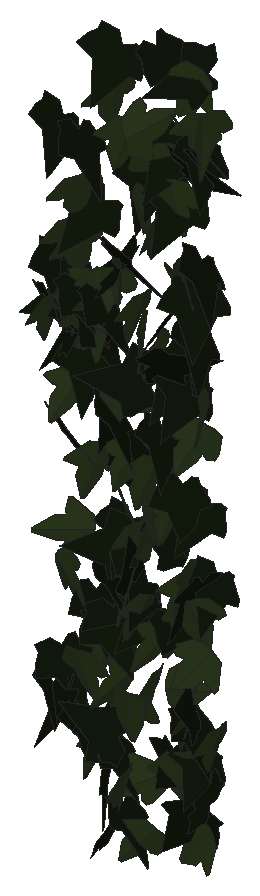
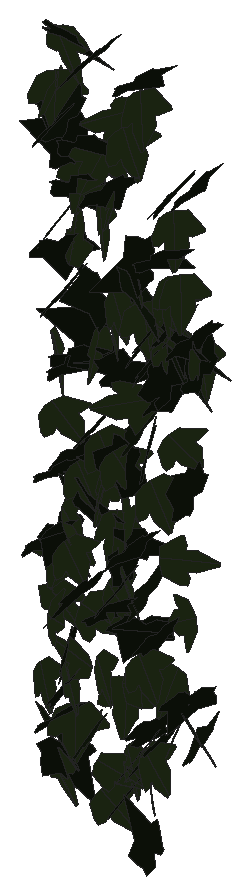
# SketchUp Ruby script. Lengths in inches.
U = 1.inch
M = Sketchup.active_model
def pt(a) = Geom::Point3d.new(a.map { |v| v * U })
def face(e, loops, mat)
  f = e.add_face(loops[0].map { |a| pt(a) })
  loops[1..].each { |l| e.add_face(l.map { |a| pt(a) }).erase! }
  f.material = f.back_material = mat if mat
  f
end
# faces: each face lists its corners as indices into pts; further lists are holes
def faces(e, pts, list, mat = nil) = list.each { |f| face(e, (f[0].is_a?(Array) ? f : [f]).map { |l| l.map { |i| pts[i] } }, mat) }
# xy, xz, yz: faces in a plane at the given z, y or x. An outline is a flat list of corners, or four numbers for a rectangle; further outlines are holes
def ring(l) = l.size == 4 ? [[l[0], l[1]], [l[2], l[1]], [l[2], l[3]], [l[0], l[3]]] : l.each_slice(2).to_a
def flat(e, list, mat, &to3) = list.each { |f| face(e, (f[0].is_a?(Array) ? f : [f]).map { |l| ring(l).map { |u, v| to3.(u, v) } }, mat) }
def xy(e, z, list, mat = nil) = flat(e, list, mat) { |x, y| [x, y, z] }
def xz(e, y, list, mat = nil) = flat(e, list, mat) { |x, z| [x, y, z] }
def yz(e, x, list, mat = nil) = flat(e, list, mat) { |y, z| [x, y, z] }
def lines(e, pts, list) = list.each { |a, b| e.add_line(pt(pts[a]), pt(pts[b])) }
# prism: a flat outline (further loops are holes) pulled along v
def prism(e, loops, v, mat = nil)
  f = face(e, loops, mat); d = Geom::Vector3d.new(v.map { |x| x * U })
  f.pushpull(f.normal.samedirection?(d) ? d.length : -d.length)
end
def box(e, o, s, mat = nil) = prism(e, [[o, [o[0] + s[0], o[1], o[2]], [o[0] + s[0], o[1] + s[1], o[2]], [o[0], o[1] + s[1], o[2]]]], [0, 0, s[2]], mat)
def at(x, y, z, deg = 0) = Geom::Transformation.translation(pt([x, y, z])) * Geom::Transformation.rotation(ORIGIN, Z_AXIS, deg.degrees)
def axes(o, x, y, z) = Geom::Transformation.new([*x, 0, *y, 0, *z, 0, *pt(o).to_a, 1])
def part(name) = M.definitions.add(name)
# library, detail: a bought-in or finely detailed component or shape, given as its bounding box
def library(name, o, s) = part(name).tap { |d| box(d.entities, o, s) }
def detail(e, o, s) = box(e.add_group.entities, o, s)
def put(e, d, t, mat = nil) = e.add_instance(d, t).tap { |i| i.material = mat if mat }
def group(e, t, mat = nil) = e.add_group.tap { |g| g.transformation = t; g.material = mat if mat }.entities
root = M.entities
M.materials.add("efeu1").color = [18, 25, 13]
M.materials.add("efeu2").color = [43, 57, 29]
c1 = part("ivyleaf_10")
p = [[0,0.5,-0.03],[-0.0625,2.02,-0.43],[-0.19,2.01,-0.46],[-0.54,1.05,-0.29],[-0.52,0.625,-0.18],[-0.83,0.76,-0.28],
  [-1.16,0.64,-0.33],[-1.15,0.33,-0.24],[-0.77,-0.39,0.02],[-0.3,-0.51,0.16],[0.04,-0.48,0.23],[-0.02,2.01,-0.4375],
  [-0.06,2.01,-0.43],[0.04,-0.49,0.23],[0.67,-0.49,0.14],[1.38,0.36,-0.2],[1.375,0.51,-0.24],[0.81,0.65,-0.19],
  [0.62,0.59,-0.15],[0.6,1.09,-0.28],[0.5,1.23,-0.31]]
faces(c1.entities,p,[[0,1,2,3,4,5,6,7,8,9,10],[11,12,0,13,14,15,16,17,18,19,20]],"efeu2")
c2 = part("ivyleaf_9")
p = [[1.54,2.16,1.25],[1.36,2.04,1.19],[-0.21,0.99,0.68],[-0.71,1.11,0.82],[-0.85,0.86,0.67],[-0.8,0.17,0.21],
  [-0.9,-0.01,0.1],[-0.67,-0.16,-0.02],[-0.08,-0.08,-0.05],[-0.03,-0.6,-0.4],[0.65,-0.88,-0.66],[0.83,-0.6,-0.49],
  [1.29,-0.42,-0.43],[1.8125,-0.07,-0.26],[1.21,0.44,0.15]]
faces(c2.entities,p,[[0,1,2,3,4,5,6,7,8,9,10,11,12,13,14]],"efeu1")
put(root,c1,axes([535.13,131.05,220.32],[0.3566,-0.77108,0.40331],[0.15176,-0.37408,-0.84937],[0.85685,0.38716,-0.01742]))
put(root,c2,axes([529.67,130.77,229.66],[-0.79255,0.50214,-0.23003],[0.19166,-0.12729,-0.93823],[-0.518,-0.81539,0.0048]))
put(root,c2,axes([529.14,130.89,212.83],[-0.83866,0.25323,-0.33738],[0.32395,-0.0943,-0.87605],[-0.2702,-0.89905,-0.00314]))
put(root,c2,axes([532.88,131.13,227.81],[-0.47309,-0.04164,0.86043],[-0.83764,-0.20693,-0.47057],[0.2011,-0.95986,0.06412]))
put(root,c1,axes([533.75,130.17,222.83],[-0.46435,0.56277,0.68264],[-0.40566,0.54969,-0.72911],[-0.78622,-0.616,-0.02698]))
put(root,c1,axes([529.6,131.16,220.19],[-0.05392,0.07152,0.95533],[-0.66511,-0.69145,0.01423],[0.68949,-0.66141,0.08843]))
put(root,c1,axes([528.33,130.79,230.19],[0.02915,-0.97812,-0.05689],[-0.00777,0.05668,-0.97854],[0.97974,0.02955,-0.00607]))
put(root,c2,axes([535.57,131.06,233],[-0.44583,-0.80919,-0.30244],[0.12747,0.275,-0.92366],[0.85441,-0.46326,-0.02002]))
put(root,c1,axes([533.64,130.37,222.18],[0.08945,-0.72433,-0.6179],[0.01533,0.62164,-0.72649],[0.95196,0.05805,0.06976]))
put(root,c1,axes([531.99,130.83,209.91],[0.21532,-0.88459,-0.06379],[-0.01557,0.06186,-0.91042],[0.88675,0.21588,-0.0005]))
put(root,c2,axes([529.45,131.52,211.5],[-0.22695,-0.167,0.97727],[-0.09236,-0.99462,-0.19141],[0.98712,-0.13145,0.20678]))
put(root,c2,axes([535.27,131.32,230.9375],[0.14126,-0.91706,0.28445],[0.04685,-0.28059,-0.92787],[0.95902,0.14879,0.00343]))
put(root,c2,axes([528.375,131.4375,238.21],[-0.08332,-0.90642,0.35778],[-0.00457,-0.35872,-0.90986],[0.97446,-0.07918,0.02633]))
put(root,c1,axes([531.47,130.8,240.9375],[-0.29212,-0.94657,-0.06972],[0.02228,0.06609,-0.99062],[0.94887,-0.29296,0.0018]))
put(root,c1,axes([534.93,130.95,232.78],[-0.88441,0.40098,0.244],[0.20352,-0.14143,0.97009],[0.42297,0.90648,0.04342]))
put(root,c2,axes([531.26,131.49,242.35],[-0.44605,-0.85808,0.25092],[0.03047,-0.29484,-0.95413],[0.89349,-0.41832,0.1578]))
put(root,c1,axes([532.97,130.54,236.36],[-0.50589,0.84599,0.13491],[-0.03905,0.13374,-0.9851],[-0.85579,-0.5062,-0.0348]))
put(root,c1,axes([533.26,131.08,224.38],[-0.32509,-0.92513,0.30258],[-0.08022,-0.29246,-0.98038],[0.97005,-0.33422,0.02033]))
put(root,c2,axes([531.1875,131.28,211.39],[-0.21397,-0.90461,-0.2182],[-0.05159,-0.21201,0.92957],[-0.92913,0.2201,-0.00137]))
put(root,c1,axes([533.05,131.07,207.6875],[-0.47987,-0.40328,0.5899],[-0.43027,-0.40424,-0.62637],[0.57051,-0.64408,0.02377]))
put(root,c2,axes([527.98,131.23,229.63],[0.28647,-0.44276,0.83663],[0.53308,-0.64684,-0.52485],[0.78218,0.603,0.05129]))
put(root,c1,axes([536.04,130.75,227.97],[0.5576,-0.85436,-0.29665],[-0.12152,0.27456,-1.01917],[0.8962,0.5688,0.04638]))
put(root,c1,axes([531.34,131.55,213.9375],[0.05294,-0.20072,0.93425],[0.17972,-0.9169,-0.20717],[0.93852,0.1869,-0.01302]))
put(root,c1,axes([530.54,130.72,229.89],[0.65262,-0.27353,-0.68758],[-0.62014,0.29804,-0.70717],[0.40375,0.89991,0.02522]))
put(root,c1,axes([532.03,131.1,239.18],[-0.44706,-0.83715,0.28329],[-0.03991,-0.29803,-0.94368],[0.88289,-0.43737,0.10079]))
put(root,c2,axes([531.92,131.12,220.2],[-0.64445,0.06946,0.66475],[-0.66835,-0.07373,-0.64024],[0.00489,-0.92292,0.10118]))
put(root,c1,axes([535.61,130.81,242.67],[0.92514,-0.16992,-0.3926],[-0.35633,0.21151,-0.93122],[0.23672,0.98248,0.13257]))
put(root,c2,axes([535.85,131.07,242.93],[-0.92387,0.19924,0.30531],[-0.31878,-0.03792,-0.93989],[-0.17689,-0.97228,0.09922]))
put(root,c1,axes([532.55,131.27,217.76],[0.07502,-0.81806,0.42556],[0.06739,-0.42096,-0.8211],[0.91967,0.09758,0.02546]))
put(root,c2,axes([533.72,130.47,229.24],[0.48356,0.58951,-0.63295],[0.39535,0.49433,0.76244],[0.76932,-0.62458,0.00603]))
put(root,c1,axes([530.01,131.04,230.4],[-0.05748,-0.96126,0.0887],[-0.00929,-0.0883,-0.96297],[0.9653,-0.05809,-0.00399]))
put(root,c2,axes([535.47,131.36,234.15],[0.26594,-0.9144,0.23622],[0.05531,-0.22991,-0.95223],[0.9428,0.27142,-0.01077]))
put(root,c2,axes([530.98,131.33,226.04],[0.43358,-0.86162,0.34254],[0.1623,-0.30177,-0.96452],[0.91289,0.46288,0.00879]))
put(root,c2,axes([531.81,131.09,208.54],[0.40908,-0.80021,-0.12614],[-0.04362,0.11935,-0.89858],[0.80892,0.41112,0.01533]))
put(root,c1,axes([529.65,130.92,235.94],[-0.38488,-0.90588,-0.08156],[0.0176,0.08113,-0.98413],[0.90938,-0.38497,-0.01548]))
put(root,c2,axes([534.56,131.27,223.74],[-0.02104,-0.94215,-0.15196],[-0.01548,0.15231,-0.94221],[0.9542,-0.01831,-0.01864]))
put(root,c1,axes([535.45,130.81,218.8],[-0.8599,-0.44619,-0.22946],[0.20327,0.10646,-0.96877],[0.45872,-0.88359,-0.00086]))
put(root,c2,axes([532.06,131.17,218.84],[0.06754,0.59082,0.71374],[-0.29613,-0.66434,0.57795],[0.87796,-0.26953,0.14003]))
put(root,c2,axes([529.64,131.4375,228.1],[-0.07839,-0.9477,0.06653],[0.0054,-0.0672,-0.95087],[0.95001,-0.07781,0.01089]))
put(root,c2,axes([535.49,131.24,219.67],[-0.26231,0.56333,-0.71902],[0.3155,-0.64617,-0.62135],[-0.85721,-0.41021,-0.00867]))
put(root,c2,axes([529.47,131,231.3],[0.41416,-0.81805,-0.35664],[-0.07895,0.35805,-0.91296],[0.88891,0.41295,0.08508]))
put(root,c1,axes([535.78,131.14,240.4],[-0.19879,0.92137,-0.36264],[-0.03134,-0.37555,-0.93698],[-0.98967,-0.17318,0.10251]))
put(root,c2,axes([534.83,131.73,213.67],[-0.05566,-0.10811,1.03495],[-0.10558,-1.03049,-0.11332],[1.03521,-0.11091,0.04409]))
put(root,c1,axes([533,130.25,239.625],[0.25234,0.03585,-1.00007],[0.45298,0.91557,0.14712],[0.89232,-0.47492,0.20813]))
put(root,c2,axes([530.59,131.43,209.83],[-0.26473,-0.01634,-0.91051],[0.88246,-0.23873,-0.25229],[-0.22486,-0.91767,0.08185]))
put(root,c1,axes([532.47,131.19,231.42],[0.05665,-0.9507,0.10335],[-0.00923,-0.10407,-0.95226],[0.95626,0.05531,-0.01532]))
put(root,c1,axes([533.51,131.59,216.64],[-0.17953,-0.62629,0.72512],[-0.16029,-0.70771,-0.65094],[0.94464,-0.23911,0.02736]))
put(root,c2,axes([535.34,131.1,209.38],[0.29123,0.30012,-0.82426],[-0.5458,-0.61791,-0.41783],[-0.68672,0.61839,-0.01748]))
put(root,c1,axes([535.71,131.12,216.53],[0.81494,-0.02544,-0.54891],[-0.54836,0.02554,-0.8153],[0.03536,0.98223,0.00698]))
put(root,c2,axes([527.76,131.64,212.28],[0.13245,-0.68718,0.55852],[0.17073,-0.53432,-0.6979],[0.86892,0.20974,0.05199]))
put(root,c1,axes([529.74,130.96,214.49],[-0.92954,0.10005,-0.136],[0.13525,-0.01428,-0.93491],[-0.10106,-0.93933,-0.00028]))
put(root,c2,axes([531.23,130.98,233.42],[0.93765,-0.33755,0.22661],[0.22032,-0.05688,-0.99634],[0.34169,0.96296,0.02058]))
put(root,c1,axes([535.84,131.02,208.5],[0.72382,-0.35821,-0.59437],[-0.5207,0.28743,-0.80732],[0.45877,0.89139,0.02147]))
put(root,c2,axes([529.49,131.24,230.71],[-0.89789,0.21157,0.39622],[-0.38438,0.09628,-0.92246],[-0.23239,-0.97669,-0.0051]))
put(root,c1,axes([534.13,131.43,222.88],[-0.35969,-0.80088,0.33456],[-0.03308,-0.34924,-0.87158],[0.86732,-0.34545,0.1055]))
put(root,c1,axes([532.36,131.52,230.26],[0.45487,-0.62548,0.53523],[0.43081,-0.34022,-0.76371],[0.7015,0.61451,0.12196]))
put(root,c2,axes([535.31,131.73,239.0625],[0.02165,-0.95056,0.25963],[0.03625,-0.25875,-0.95036],[0.98472,0.03043,0.02927]))
put(root,c1,axes([533.33,131.09,235.3],[0.3168,-0.8909,-0.24909],[-0.02647,0.25445,-0.94375],[0.92469,0.31251,0.05832]))
put(root,c2,axes([530.1875,131.22,229.88],[0.45021,-0.79874,-0.27058],[-0.09574,0.25633,-0.91598],[0.83788,0.45847,0.04072]))
put(root,c2,axes([534.72,131.29,238.2],[0.53872,-0.32013,0.77885],[0.68328,-0.37422,-0.62642],[0.49217,0.86994,0.01714]))
put(root,c1,axes([530.27,131.29,231.17],[0.5007,0.03023,-0.87991],[-0.87964,-0.02576,-0.50143],[-0.03735,1.01207,0.01352]))
put(root,c2,axes([534.6,131.87,228.05],[-0.38959,-0.81672,0.31633],[-0.07913,-0.31198,-0.90293],[0.87226,-0.39308,0.05938]))
put(root,c1,axes([531.71,131.51,218.6],[0.65513,-0.70743,0.27215],[0.15949,-0.223,-0.96361],[0.741,0.67344,-0.0332]))
put(root,c2,axes([529.26,131.45,237.81],[0.33741,-0.92031,-0.08279],[0.01487,0.09354,-0.97914],[0.92391,0.33459,0.04599]))
put(root,c2,axes([533.2,131.76,225.52],[0.07275,-0.89281,0.30246],[0.05848,-0.2985,-0.89519],[0.94084,0.08759,0.03226]))
put(root,c1,axes([531.61,131.61,221.03],[-0.50387,0.23543,0.8566],[0.73119,-0.4494,0.55361],[0.50454,0.88639,0.05316]))
put(root,c2,axes([534.82,131.58,239.42],[0.38343,-0.62183,0.667],[0.5112,-0.45261,-0.71583],[0.75514,0.62214,0.14591]))
put(root,c2,axes([536.15,130.875,210.16],[-0.49571,0.65477,0.44064],[-0.27846,0.34179,-0.82113],[-0.73848,-0.5684,0.01384]))
put(root,c2,axes([530.89,131.31,216.71],[-0.16959,-0.69626,-0.56872],[0.28055,0.50886,-0.70663],[0.85411,-0.30539,0.11919]))
put(root,c2,axes([534.7,131.04,221.33],[-0.48403,0.32589,0.79539],[-0.66443,0.43727,-0.58349],[-0.54534,-0.82203,0.00495]))
put(root,c1,axes([535.68,131.27,240.64],[-0.63456,-0.76366,-0.01621],[0.03227,-0.00575,-0.99249],[0.76315,-0.63474,0.02849]))
put(root,c2,axes([530.33,131.26,231.04],[0.50401,-0.77526,-0.34102],[-0.14642,0.3111,-0.92365],[0.83419,0.52301,0.04392]))
put(root,c1,axes([532.01,131.21,213.27],[-1.00429,-0.14144,0.13334],[-0.13107,-0.02543,-1.01417],[0.14355,-1.01278,0.00685]))
put(root,c2,axes([530.5,131.64,218.43],[0.43644,-0.75539,0.27806],[0.16591,-0.2251,-0.8719],[0.78766,0.46597,0.02957]))
put(root,c1,axes([534.04,131.28,236.97],[-0.97594,-0.06903,-0.18062],[0.18829,-0.12778,-0.96854],[0.04401,-0.98425,0.13841]))
put(root,c1,axes([528.39,131.55,218.04],[-0.45735,0.28616,-0.77799],[0.61911,-0.47295,-0.53791],[-0.55124,-0.76861,0.04134]))
put(root,c2,axes([535.21,131.99,222.84],[-0.4686,-0.73714,0.27454],[0.02248,-0.33198,-0.853],[0.78628,-0.42982,0.18801]))
put(root,c2,axes([530.22,132,225.38],[0.28309,-0.34009,-0.9045],[0.81161,-0.42787,0.41489],[-0.52447,-0.84568,0.15383]))
put(root,c2,axes([534.35,131.82,236.59],[-0.76798,-0.59788,-0.03979],[0.03966,0.01383,-0.97317],[0.59789,-0.76888,0.01344]))
put(root,c1,axes([528.83,131.85,226.28],[-0.45699,-0.55016,0.61285],[-0.08479,-0.66572,-0.66085],[0.81919,-0.37582,0.27348]))
put(root,c2,axes([534,130.5625,231.03],[-0.42591,0.70136,-0.55817],[-0.28653,0.47903,0.82055],[0.84933,0.51331,-0.00308]))
put(root,c2,axes([529.34,131.62,228.83],[0.82592,-0.00109,-0.48629],[0.48625,0.01365,0.82583],[0.00599,-0.95835,0.01231]))
put(root,c1,axes([531.45,131.15,232.37],[0.59346,-0.6578,-0.38916],[-0.06497,0.44751,-0.85549],[0.76153,0.5508,0.23029]))
put(root,c2,axes([529.87,132.05,234.65],[-0.63416,-0.67483,0.27106],[-0.06625,-0.30454,-0.91317],[0.72421,-0.61877,0.15382]))
put(root,c2,axes([530.08,131.13,211.59],[0.50811,-0.53307,-0.51418],[-0.17983,0.5161,-0.71276],[0.71848,0.50617,0.18523]))
put(root,c2,axes([531,131.47,216.875],[-0.25497,-0.71747,-0.56983],[0.22414,0.52467,-0.7609],[0.88839,-0.33829,0.02843]))
put(root,c2,axes([530.87,131.49,210.89],[0.44966,-0.75577,-0.17635],[-0.06178,0.1683,-0.87883],[0.77361,0.45273,0.03231]))
put(root,c2,axes([528.4,131.4375,214.29],[0.01709,-0.75885,-0.49143],[0.05919,0.4914,-0.75674],[0.90213,-0.01787,0.05896]))
put(root,c1,axes([534.51,131.77,219.15],[-0.28005,-0.81154,0.37848],[0.02065,-0.4023,-0.84734],[0.89522,-0.24459,0.13795]))
put(root,c1,axes([531.86,131.82,224.33],[-0.47537,-0.67383,0.50305],[-0.11741,-0.51903,-0.80617],[0.83266,-0.45788,0.17352]))
put(root,c1,axes([529.34,131.34,233.16],[-0.32406,-0.89566,-0.18955],[0.06286,0.17883,-0.95248],[0.91334,-0.3301,-0.0017]))
put(root,c1,axes([530.02,131.74,223.52],[-0.38833,-0.86947,0.34539],[-0.04676,-0.35546,-0.94739],[0.93439,-0.37914,0.09613]))
put(root,c2,axes([528.07,131.77,224.04],[0.48169,-0.5274,0.64224],[0.4492,-0.45931,-0.71408],[0.69918,0.65844,0.01631]))
put(root,c2,axes([533.43,132.16,210.55],[-0.15451,-0.50177,0.73344],[0.06536,-0.74884,-0.49854],[0.88625,-0.03225,0.16464]))
put(root,c1,axes([530.15,131.83,210.85],[0.04007,-0.89822,0.35868],[0.00189,-0.35891,-0.89902],[0.96719,0.03791,-0.0131]))
put(root,c1,axes([531.31,131.22,227.1],[-0.28816,-0.16345,-0.97247],[0.95599,0.20218,-0.31726],[0.24185,-0.99391,0.09539]))
put(root,c1,axes([533.18,131.32,238.22],[-0.85945,-0.35297,-0.36931],[0.35638,0.10361,-0.92839],[0.36602,-0.92969,0.03675]))
put(root,c1,axes([532.34,131.38,221.11],[-0.32323,-0.84869,-0.22259],[0.09579,0.20166,-0.90799],[0.87215,-0.33668,0.01723]))
put(root,c1,axes([532.52,131.81,209.69],[-0.40117,-0.01536,0.76306],[-0.59347,-0.53575,-0.32279],[0.47989,-0.6754,0.2387]))
put(root,c1,axes([534.42,131.5,211.3],[-0.7155,-0.68219,0.02217],[-0.0072,-0.02457,-0.98851],[0.68252,-0.71542,0.01281]))
put(root,c2,axes([533.88,131.98,238.7],[-0.80098,-0.55514,-0.05475],[0.0407,0.03739,-0.97452],[0.55634,-0.80198,-0.00753]))
put(root,c1,axes([528.83,131.51,233.49],[-0.36958,-0.89227,-0.08847],[0.02102,0.08704,-0.96568],[0.8964,-0.36992,-0.01383]))
put(root,c2,axes([531.9375,132.25,218.07],[-0.0616,-0.77135,0.55593],[0.016,-0.55785,-0.77226],[0.95068,-0.0406,0.04902]))
put(root,c2,axes([532.49,132.23,217.12],[-0.51344,-0.64008,0.39025],[-0.11095,-0.40291,-0.80683],[0.74141,-0.50356,0.14951]))
put(root,c2,axes([532.48,132.09,237.05],[-0.32531,-0.91086,0.06434],[0.0027,-0.06926,-0.96686],[0.91313,-0.3243,0.02579]))
put(root,c2,axes([530.45,131.39,206.27],[0.07239,0.87428,0.34753],[-0.08393,-0.34116,0.87576],[0.93707,-0.0981,0.05159]))
put(root,c2,axes([533.25,131.39,243.03],[0.54507,-0.70362,-0.44634],[-0.04498,0.50774,-0.85532],[0.83203,0.48839,0.24617]))
put(root,c1,axes([535.9375,131.66,212.89],[0.08536,-0.87572,0.01385],[0.00495,-0.01344,-0.87987],[0.87582,0.08542,0.00362]))
put(root,c1,axes([530.63,131.71,231.66],[-0.62971,-0.72269,0.15139],[-0.01859,-0.18339,-0.95276],[0.73814,-0.62114,0.10516]))
put(root,c2,axes([531.49,131.17,232.53],[-0.42377,0.81762,0.32765],[-0.22266,0.25236,-0.9177],[-0.85222,-0.4725,0.07684]))
put(root,c2,axes([534.17,132.16,228.72],[-0.67311,-0.67117,0.11029],[-0.02019,-0.13538,-0.94708],[0.67987,-0.66851,0.08107]))
put(root,c2,axes([527.9,132.03,231.6],[-0.04243,-0.94644,0.00236],[-0.00652,-0.00207,-0.94737],[0.94642,-0.04245,-0.00642]))
put(root,c1,axes([532.78,131.8,214.3],[0.26947,-0.86458,0.10976],[0.04386,-0.10129,-0.90552],[0.87041,0.27277,0.01165]))
put(root,c2,axes([534.93,132.2,211.34],[-0.29634,-0.78994,0.22667],[0.04034,-0.25465,-0.8347],[0.82082,-0.27267,0.12286]))
put(root,c2,axes([533.9,131.43,217.68],[0.4989,-0.68449,-0.52478],[-0.10359,0.55431,-0.82148],[0.85627,0.46587,0.20638]))
put(root,c2,axes([535.54,132.19,219.63],[-0.20568,-0.87645,0.17192],[-0.01105,-0.1739,-0.89981],[0.89308,-0.204,0.02846]))
put(root,c1,axes([534.55,131.76,213.45],[0.27558,-0.90268,-0.01144],[-0.00351,0.01089,-0.94381],[0.90275,0.2756,-0.00018]))
put(root,c2,axes([531.375,131.52,224.21],[0.35511,-0.02501,-0.89925],[0.73882,0.55968,0.27619],[0.51325,-0.78836,0.22461]))
put(root,c1,axes([533.17,131.4375,229.53],[0.1501,-0.83511,-0.40447],[0.15013,0.42619,-0.82423],[0.91568,0.06702,0.20144]))
put(root,c2,axes([529.69,131.95,217],[0.1139,-0.89327,-0.14883],[-0.01915,0.14759,-0.9005],[0.90538,0.11549,-0.00032]))
put(root,c2,axes([531.1,132.29,220.59],[-0.20177,-0.86159,0.25274],[-0.00107,-0.25881,-0.88314],[0.89789,-0.19392,0.05574]))
put(root,c2,axes([534.43,131.87,213.1],[0.3456,-0.8414,-0.15455],[-0.04706,0.14773,-0.90953],[0.85418,0.34857,0.01242]))
put(root,c1,axes([534.82,132.12,225.83],[-0.60417,-0.50426,0.53331],[-0.16498,-0.57978,-0.73509],[0.71518,-0.55973,0.28096]))
put(root,c1,axes([533.83,131.8125,214.22],[0.22425,-0.15758,-0.89109],[0.85543,-0.2625,0.2617],[-0.29513,-0.88058,0.08145]))
put(root,c1,axes([530.41,132.04,215.33],[-0.3146,-0.83352,0.29326],[-0.02902,-0.30138,-0.88773],[0.88313,-0.30683,0.0753]))
put(root,c1,axes([534.92,132.34,216.14],[0.17282,-0.51553,0.74616],[0.44596,-0.61311,-0.5269],[0.78972,0.45904,0.13425]))
